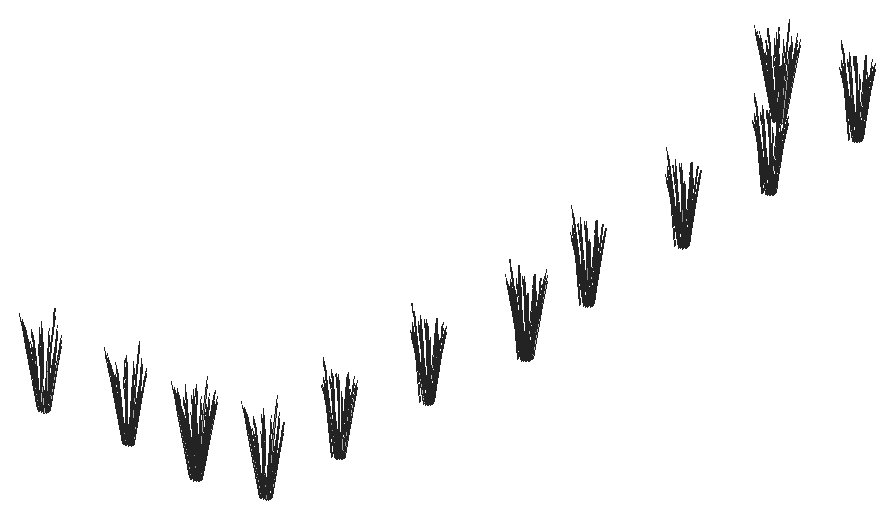
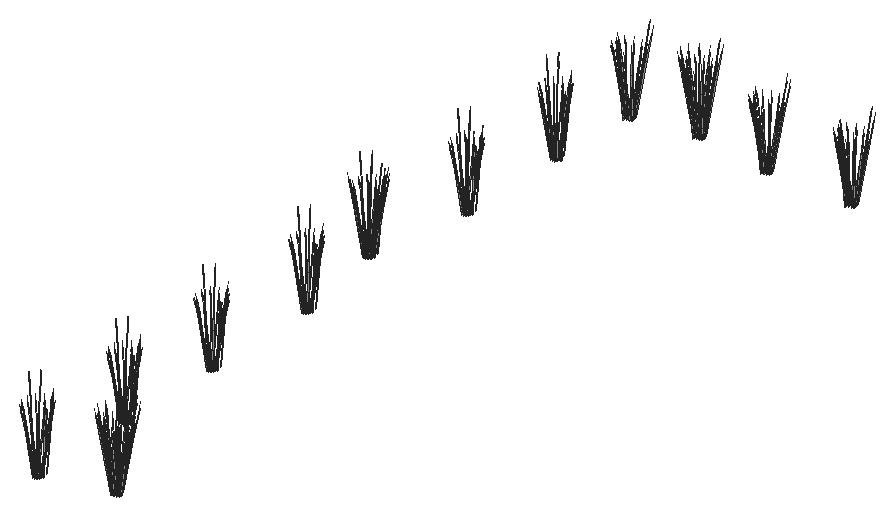
# SketchUp Ruby script. Lengths in inches.
U = 1.inch
M = Sketchup.active_model
def pt(a) = Geom::Point3d.new(a.map { |v| v * U })
def face(e, loops, mat)
  f = e.add_face(loops[0].map { |a| pt(a) })
  loops[1..].each { |l| e.add_face(l.map { |a| pt(a) }).erase! }
  f.material = f.back_material = mat if mat
  f
end
# faces: each face lists its corners as indices into pts; further lists are holes
def faces(e, pts, list, mat = nil) = list.each { |f| face(e, (f[0].is_a?(Array) ? f : [f]).map { |l| l.map { |i| pts[i] } }, mat) }
# xy, xz, yz: faces in a plane at the given z, y or x. An outline is a flat list of corners, or four numbers for a rectangle; further outlines are holes
def ring(l) = l.size == 4 ? [[l[0], l[1]], [l[2], l[1]], [l[2], l[3]], [l[0], l[3]]] : l.each_slice(2).to_a
def flat(e, list, mat, &to3) = list.each { |f| face(e, (f[0].is_a?(Array) ? f : [f]).map { |l| ring(l).map { |u, v| to3.(u, v) } }, mat) }
def xy(e, z, list, mat = nil) = flat(e, list, mat) { |x, y| [x, y, z] }
def xz(e, y, list, mat = nil) = flat(e, list, mat) { |x, z| [x, y, z] }
def yz(e, x, list, mat = nil) = flat(e, list, mat) { |y, z| [x, y, z] }
def lines(e, pts, list) = list.each { |a, b| e.add_line(pt(pts[a]), pt(pts[b])) }
# prism: a flat outline (further loops are holes) pulled along v
def prism(e, loops, v, mat = nil)
  f = face(e, loops, mat); d = Geom::Vector3d.new(v.map { |x| x * U })
  f.pushpull(f.normal.samedirection?(d) ? d.length : -d.length)
end
def box(e, o, s, mat = nil) = prism(e, [[o, [o[0] + s[0], o[1], o[2]], [o[0] + s[0], o[1] + s[1], o[2]], [o[0], o[1] + s[1], o[2]]]], [0, 0, s[2]], mat)
def at(x, y, z, deg = 0) = Geom::Transformation.translation(pt([x, y, z])) * Geom::Transformation.rotation(ORIGIN, Z_AXIS, deg.degrees)
def axes(o, x, y, z) = Geom::Transformation.new([*x, 0, *y, 0, *z, 0, *pt(o).to_a, 1])
def part(name) = M.definitions.add(name)
# library, detail: a bought-in or finely detailed component or shape, given as its bounding box
def library(name, o, s) = part(name).tap { |d| box(d.entities, o, s) }
def detail(e, o, s) = box(e.add_group.entities, o, s)
def put(e, d, t, mat = nil) = e.add_instance(d, t).tap { |i| i.material = mat if mat }
def group(e, t, mat = nil) = e.add_group.tap { |g| g.transformation = t; g.material = mat if mat }.entities
root = M.entities
M.materials.add("LightPink_Translucent").color = [175, 214, 192]
M.materials["LightPink_Translucent"].alpha = 0.75
c1 = part("blade")
p = [[2.15,0.21,22],[0,0.17,0],[0.09,0.45,0],[2.18,0.31,22],[2.29,0.31,22],[0.38,0.45,0],
  [2.48,0.24,33],[2.49,0.24,33],[2.48,0.22,33]]
faces(c1.entities,p,[[0,1,2,3],[4,5,2,3],[6,3,4,7],[8,0,3,6]])
c2 = part("seeds")
p = [[0.3,-0.1,1.38],[-0.01,-0.03,1.59],[-0.01,-0.03,0.03],[0.14,-0.07,-0.07],[0.29,-0.03,3],[0.15,0.01,3.11]]
faces(c2.entities,p,[[0,1,2,3],[1,0,4,5]],"LightPink_Translucent")
c3 = part("blade with seeds")
put(c3.entities,c1,at(0,0,0))
put(c3.entities,c2,axes([2.4,0.25,30.99],[1.5799,-0.05474,1.17369],[-0.12525,1.92788,0.29478],[-0.07173,-0.02425,1.56792]))
put(root,c3,axes([499.79,369.26,141.57],[0.40986,-0.11853,0.43682],[0.07113,0.46497,0.36018],[-0.09639,-0.13704,0.9039]))
put(root,c3,axes([498.96,369.9375,141.57],[0.30385,-0.34034,0.43682],[0.26205,0.36143,0.36018],[-0.14256,-0.06278,0.9039]))
put(root,c3,axes([501.97,372.85,141.57],[-0.30385,0.34034,0.43682],[-0.26205,-0.36143,0.36018],[0.14256,0.06278,0.9039]))
put(root,c3,axes([500.8,369.15,141.57],[0.40605,0.13503,0.43682],[-0.13885,0.44393,0.36018],[-0.0244,-0.17458,0.9039]))
put(root,c3,axes([501.14,373.53,141.57],[-0.40986,0.11853,0.43682],[-0.07113,-0.46497,0.36018],[0.09639,0.13704,0.9039]))
put(root,c3,axes([498.625,372.18,141.57],[-0.1022,-0.47536,0.43682],[0.4009,-0.0825,0.36018],[-0.11815,0.1118,0.9039]))
put(root,c3,axes([463.68,229.6,141.57],[0.47094,0.11642,0.43682],[-0.16104,0.38276,0.36018],[-0.0283,-0.15052,0.9039]))
put(root,c3,axes([465.05,232.79,141.57],[-0.35241,0.29344,0.43682],[-0.30393,-0.31162,0.36018],[0.16534,0.05413,0.9039]))
put(root,c3,axes([465.54,231.87,141.57],[-0.13503,0.40605,0.43682],[-0.44393,-0.13885,0.36018],[0.17458,-0.0244,0.9039]))
put(root,c3,axes([461.16,232.21,141.57],[-0.11853,-0.40986,0.43682],[0.46497,-0.07113,0.36018],[-0.13704,0.09639,0.9039]))
put(root,c3,axes([461.84,233.04,141.57],[-0.34034,-0.30385,0.43682],[0.36143,-0.26205,0.36018],[-0.06278,0.14256,0.9039]))
put(root,c3,axes([464.75,230.03,141.57],[0.34034,0.30385,0.43682],[-0.36143,0.26205,0.36018],[0.06278,-0.14256,0.9039]))
put(root,c3,axes([461.06,231.2,141.57],[0.13503,-0.40605,0.43682],[0.44393,0.13885,0.36018],[-0.17458,0.0244,0.9039]))
put(root,c3,axes([465.43,230.86,141.57],[0.11853,0.40986,0.43682],[-0.46497,0.07113,0.36018],[0.13704,-0.09639,0.9039]))
put(root,c3,axes([464.08,233.375,141.57],[-0.47536,0.1022,0.43682],[-0.0825,-0.4009,0.36018],[0.1118,0.11815,0.9039]))
put(root,c3,axes([463.68,558.11,141.57],[0.47094,0.11642,0.43682],[-0.16104,0.38276,0.36018],[-0.0283,-0.15052,0.9039]))
put(root,c3,axes([465.05,561.3,141.57],[-0.35241,0.29344,0.43682],[-0.30393,-0.31162,0.36018],[0.16534,0.05413,0.9039]))
put(root,c3,axes([465.54,560.38,141.57],[-0.13503,0.40605,0.43682],[-0.44393,-0.13885,0.36018],[0.17458,-0.0244,0.9039]))
put(root,c3,axes([461.16,560.73,141.57],[-0.11853,-0.40986,0.43682],[0.46497,-0.07113,0.36018],[-0.13704,0.09639,0.9039]))
put(root,c3,axes([461.84,561.56,141.57],[-0.34034,-0.30385,0.43682],[0.36143,-0.26205,0.36018],[-0.06278,0.14256,0.9039]))
put(root,c3,axes([464.75,558.54,141.57],[0.34034,0.30385,0.43682],[-0.36143,0.26205,0.36018],[0.06278,-0.14256,0.9039]))
put(root,c3,axes([461.06,559.71,141.57],[0.13503,-0.40605,0.43682],[0.44393,0.13885,0.36018],[-0.17458,0.0244,0.9039]))
put(root,c3,axes([465.43,559.37,141.57],[0.11853,0.40986,0.43682],[-0.46497,0.07113,0.36018],[0.13704,-0.09639,0.9039]))
put(root,c3,axes([464.08,561.89,141.57],[-0.47536,0.1022,0.43682],[-0.0825,-0.4009,0.36018],[0.1118,0.11815,0.9039]))
put(root,c3,axes([390.43,238,141.77],[0.14409,-0.34247,0.32227],[0.42037,0.09989,-0.41605],[0.03855,0.13788,0.79608]))
put(root,c3,axes([391.2,234.7,141.77],[-0.14409,0.34247,0.32227],[-0.42037,-0.09989,-0.41605],[-0.03855,-0.13788,0.79608]))
put(root,c3,axes([392.28,237.46,141.77],[-0.27194,-0.27882,0.32227],[0.31051,-0.26394,-0.41605],[0.15777,0.04016,0.79608]))
put(root,c3,axes([392.73,236.68,141.77],[-0.3972,-0.12423,0.32227],[0.11585,-0.36244,-0.41605],[0.15992,-0.03323,0.79608]))
put(root,c3,axes([389.35,235.24,141.77],[0.27194,0.27882,0.32227],[-0.31051,0.26394,-0.41605],[-0.15777,-0.04016,0.79608]))
put(root,c3,axes([389.53,237.62,141.77],[0.32338,-0.23447,0.32227],[0.30612,0.26773,-0.41605],[-0.04658,0.13603,0.79608]))
put(root,c3,axes([388.97,236.89,141.77],[0.41603,-0.06364,0.32227],[0.10985,0.36383,-0.41605],[-0.11922,0.09772,0.79608]))
put(root,c3,axes([391.44,237.95,141.77],[-0.07382,-0.3587,0.32227],[0.42197,-0.09472,-0.41605],[0.11334,0.10279,0.79608]))
put(root,c3,axes([392.67,235.8125,141.77],[-0.41603,0.06364,0.32227],[-0.10985,-0.36383,-0.41605],[0.11922,-0.09772,0.79608]))
put(root,c3,axes([388.9,236.02,141.77],[0.3972,0.12423,0.32227],[-0.11585,0.36244,-0.41605],[-0.15992,0.03323,0.79608]))
put(root,c3,axes([392.1,235.09,141.77],[-0.32338,0.23447,0.32227],[-0.30612,-0.26773,-0.41605],[0.04658,-0.13603,0.79608]))
put(root,c3,axes([390.1875,234.76,141.77],[0.07382,0.3587,0.32227],[-0.42197,0.09472,-0.41605],[-0.11334,-0.10279,0.79608]))
put(root,c3,axes([428.63,238,141.77],[0.14409,-0.34247,0.32227],[0.42037,0.09989,-0.41605],[0.03855,0.13788,0.79608]))
put(root,c3,axes([429.39,234.7,141.77],[-0.14409,0.34247,0.32227],[-0.42037,-0.09989,-0.41605],[-0.03855,-0.13788,0.79608]))
put(root,c3,axes([430.48,237.46,141.77],[-0.27194,-0.27882,0.32227],[0.31051,-0.26394,-0.41605],[0.15777,0.04016,0.79608]))
put(root,c3,axes([430.93,236.68,141.77],[-0.3972,-0.12423,0.32227],[0.11585,-0.36244,-0.41605],[0.15992,-0.03323,0.79608]))
put(root,c3,axes([427.54,235.24,141.77],[0.27194,0.27882,0.32227],[-0.31051,0.26394,-0.41605],[-0.15777,-0.04016,0.79608]))
put(root,c3,axes([427.72,237.62,141.77],[0.32338,-0.23447,0.32227],[0.30612,0.26773,-0.41605],[-0.04658,0.13603,0.79608]))
put(root,c3,axes([427.16,236.89,141.77],[0.41603,-0.06364,0.32227],[0.10985,0.36383,-0.41605],[-0.11922,0.09772,0.79608]))
put(root,c3,axes([429.64,237.95,141.77],[-0.07382,-0.3587,0.32227],[0.42197,-0.09472,-0.41605],[0.11334,0.10279,0.79608]))
put(root,c3,axes([430.86,235.8125,141.77],[-0.41603,0.06364,0.32227],[-0.10985,-0.36383,-0.41605],[0.11922,-0.09772,0.79608]))
put(root,c3,axes([427.09,236.02,141.77],[0.3972,0.12423,0.32227],[-0.11585,0.36244,-0.41605],[-0.15992,0.03323,0.79608]))
put(root,c3,axes([430.3,235.09,141.77],[-0.32338,0.23447,0.32227],[-0.30612,-0.26773,-0.41605],[0.04658,-0.13603,0.79608]))
put(root,c3,axes([428.38,234.76,141.77],[0.07382,0.3587,0.32227],[-0.42197,0.09472,-0.41605],[-0.11334,-0.10279,0.79608]))
put(root,c3,axes([490.64,238,141.77],[0.14409,-0.34247,0.32227],[0.42037,0.09989,-0.41605],[0.03855,0.13788,0.79608]))
put(root,c3,axes([491.4,234.7,141.77],[-0.14409,0.34247,0.32227],[-0.42037,-0.09989,-0.41605],[-0.03855,-0.13788,0.79608]))
put(root,c3,axes([492.49,237.46,141.77],[-0.27194,-0.27882,0.32227],[0.31051,-0.26394,-0.41605],[0.15777,0.04016,0.79608]))
put(root,c3,axes([492.9375,236.68,141.77],[-0.3972,-0.12423,0.32227],[0.11585,-0.36244,-0.41605],[0.15992,-0.03323,0.79608]))
put(root,c3,axes([489.55,235.24,141.77],[0.27194,0.27882,0.32227],[-0.31051,0.26394,-0.41605],[-0.15777,-0.04016,0.79608]))
put(root,c3,axes([489.73,237.62,141.77],[0.32338,-0.23447,0.32227],[0.30612,0.26773,-0.41605],[-0.04658,0.13603,0.79608]))
put(root,c3,axes([489.17,236.89,141.77],[0.41603,-0.06364,0.32227],[0.10985,0.36383,-0.41605],[-0.11922,0.09772,0.79608]))
put(root,c3,axes([491.65,237.95,141.77],[-0.07382,-0.3587,0.32227],[0.42197,-0.09472,-0.41605],[0.11334,0.10279,0.79608]))
put(root,c3,axes([492.87,235.8125,141.77],[-0.41603,0.06364,0.32227],[-0.10985,-0.36383,-0.41605],[0.11922,-0.09772,0.79608]))
put(root,c3,axes([489.11,236.02,141.77],[0.3972,0.12423,0.32227],[-0.11585,0.36244,-0.41605],[-0.15992,0.03323,0.79608]))
put(root,c3,axes([492.31,235.09,141.77],[-0.32338,0.23447,0.32227],[-0.30612,-0.26773,-0.41605],[0.04658,-0.13603,0.79608]))
put(root,c3,axes([490.39,234.76,141.77],[0.07382,0.3587,0.32227],[-0.42197,0.09472,-0.41605],[-0.11334,-0.10279,0.79608]))
put(root,c3,axes([491.37,275.12,141.77],[0.34247,0.14409,0.32227],[-0.09989,0.42037,-0.41605],[-0.13788,0.03855,0.79608]))
put(root,c3,axes([494.67,275.88,141.77],[-0.34247,-0.14409,0.32227],[0.09989,-0.42037,-0.41605],[0.13788,-0.03855,0.79608]))
put(root,c3,axes([491.91,276.97,141.77],[0.27882,-0.27194,0.32227],[0.26394,0.31051,-0.41605],[-0.04016,0.15777,0.79608]))
put(root,c3,axes([492.69,277.42,141.77],[0.12423,-0.3972,0.32227],[0.36244,0.11585,-0.41605],[0.03323,0.15992,0.79608]))
put(root,c3,axes([494.13,274.03,141.77],[-0.27882,0.27194,0.32227],[-0.26394,-0.31051,-0.41605],[0.04016,-0.15777,0.79608]))
put(root,c3,axes([491.76,274.21,141.77],[0.23447,0.32338,0.32227],[-0.26773,0.30612,-0.41605],[-0.13603,-0.04658,0.79608]))
put(root,c3,axes([492.48,273.65,141.77],[0.06364,0.41603,0.32227],[-0.36383,0.10985,-0.41605],[-0.09772,-0.11922,0.79608]))
put(root,c3,axes([491.43,276.13,141.77],[0.3587,-0.07382,0.32227],[0.09472,0.42197,-0.41605],[-0.10279,0.11334,0.79608]))
put(root,c3,axes([493.5625,277.35,141.77],[-0.06364,-0.41603,0.32227],[0.36383,-0.10985,-0.41605],[0.09772,0.11922,0.79608]))
put(root,c3,axes([493.35,273.59,141.77],[-0.12423,0.3972,0.32227],[-0.36244,-0.11585,-0.41605],[-0.03323,-0.15992,0.79608]))
put(root,c3,axes([494.29,276.79,141.77],[-0.23447,-0.32338,0.32227],[0.26773,-0.30612,-0.41605],[0.13603,0.04658,0.79608]))
put(root,c3,axes([494.62,274.875,141.77],[-0.3587,0.07382,0.32227],[-0.09472,-0.42197,-0.41605],[0.10279,-0.11334,0.79608]))
put(root,c3,axes([491.37,325.11,141.77],[0.34247,0.14409,0.32227],[-0.09989,0.42037,-0.41605],[-0.13788,0.03855,0.79608]))
put(root,c3,axes([494.67,325.87,141.77],[-0.34247,-0.14409,0.32227],[0.09989,-0.42037,-0.41605],[0.13788,-0.03855,0.79608]))
put(root,c3,axes([491.91,326.96,141.77],[0.27882,-0.27194,0.32227],[0.26394,0.31051,-0.41605],[-0.04016,0.15777,0.79608]))
put(root,c3,axes([492.69,327.4,141.77],[0.12423,-0.3972,0.32227],[0.36244,0.11585,-0.41605],[0.03323,0.15992,0.79608]))
put(root,c3,axes([494.13,324.02,141.77],[-0.27882,0.27194,0.32227],[-0.26394,-0.31051,-0.41605],[0.04016,-0.15777,0.79608]))
put(root,c3,axes([491.76,324.2,141.77],[0.23447,0.32338,0.32227],[-0.26773,0.30612,-0.41605],[-0.13603,-0.04658,0.79608]))
put(root,c3,axes([492.48,323.64,141.77],[0.06364,0.41603,0.32227],[-0.36383,0.10985,-0.41605],[-0.09772,-0.11922,0.79608]))
put(root,c3,axes([491.43,326.12,141.77],[0.3587,-0.07382,0.32227],[0.09472,0.42197,-0.41605],[-0.10279,0.11334,0.79608]))
put(root,c3,axes([493.5625,327.34,141.77],[-0.06364,-0.41603,0.32227],[0.36383,-0.10985,-0.41605],[0.09772,0.11922,0.79608]))
put(root,c3,axes([493.35,323.57,141.77],[-0.12423,0.3972,0.32227],[-0.36244,-0.11585,-0.41605],[-0.03323,-0.15992,0.79608]))
put(root,c3,axes([494.29,326.78,141.77],[-0.23447,-0.32338,0.32227],[0.26773,-0.30612,-0.41605],[0.13603,0.04658,0.79608]))
put(root,c3,axes([494.62,324.86,141.77],[-0.3587,0.07382,0.32227],[-0.09472,-0.42197,-0.41605],[0.10279,-0.11334,0.79608]))
put(root,c3,axes([491.37,415.23,141.77],[0.34247,0.14409,0.32227],[-0.09989,0.42037,-0.41605],[-0.13788,0.03855,0.79608]))
put(root,c3,axes([494.67,415.99,141.77],[-0.34247,-0.14409,0.32227],[0.09989,-0.42037,-0.41605],[0.13788,-0.03855,0.79608]))
put(root,c3,axes([491.91,417.08,141.77],[0.27882,-0.27194,0.32227],[0.26394,0.31051,-0.41605],[-0.04016,0.15777,0.79608]))
put(root,c3,axes([492.69,417.52,141.77],[0.12423,-0.3972,0.32227],[0.36244,0.11585,-0.41605],[0.03323,0.15992,0.79608]))
put(root,c3,axes([494.13,414.14,141.77],[-0.27882,0.27194,0.32227],[-0.26394,-0.31051,-0.41605],[0.04016,-0.15777,0.79608]))
put(root,c3,axes([491.76,414.32,141.77],[0.23447,0.32338,0.32227],[-0.26773,0.30612,-0.41605],[-0.13603,-0.04658,0.79608]))
put(root,c3,axes([492.48,413.76,141.77],[0.06364,0.41603,0.32227],[-0.36383,0.10985,-0.41605],[-0.09772,-0.11922,0.79608]))
put(root,c3,axes([491.43,416.24,141.77],[0.3587,-0.07382,0.32227],[0.09472,0.42197,-0.41605],[-0.10279,0.11334,0.79608]))
put(root,c3,axes([493.5625,417.46,141.77],[-0.06364,-0.41603,0.32227],[0.36383,-0.10985,-0.41605],[0.09772,0.11922,0.79608]))
put(root,c3,axes([493.35,413.69,141.77],[-0.12423,0.3972,0.32227],[-0.36244,-0.11585,-0.41605],[-0.03323,-0.15992,0.79608]))
put(root,c3,axes([494.29,416.9,141.77],[-0.23447,-0.32338,0.32227],[0.26773,-0.30612,-0.41605],[0.13603,0.04658,0.79608]))
put(root,c3,axes([494.62,414.98,141.77],[-0.3587,0.07382,0.32227],[-0.09472,-0.42197,-0.41605],[0.10279,-0.11334,0.79608]))
put(root,c3,axes([491.37,468.8,141.77],[0.34247,0.14409,0.32227],[-0.09989,0.42037,-0.41605],[-0.13788,0.03855,0.79608]))
put(root,c3,axes([494.67,469.5625,141.77],[-0.34247,-0.14409,0.32227],[0.09989,-0.42037,-0.41605],[0.13788,-0.03855,0.79608]))
put(root,c3,axes([491.91,470.65,141.77],[0.27882,-0.27194,0.32227],[0.26394,0.31051,-0.41605],[-0.04016,0.15777,0.79608]))
put(root,c3,axes([492.69,471.1,141.77],[0.12423,-0.3972,0.32227],[0.36244,0.11585,-0.41605],[0.03323,0.15992,0.79608]))
put(root,c3,axes([494.13,467.71,141.77],[-0.27882,0.27194,0.32227],[-0.26394,-0.31051,-0.41605],[0.04016,-0.15777,0.79608]))
put(root,c3,axes([491.76,467.89,141.77],[0.23447,0.32338,0.32227],[-0.26773,0.30612,-0.41605],[-0.13603,-0.04658,0.79608]))
put(root,c3,axes([492.48,467.33,141.77],[0.06364,0.41603,0.32227],[-0.36383,0.10985,-0.41605],[-0.09772,-0.11922,0.79608]))
put(root,c3,axes([491.43,469.81,141.77],[0.3587,-0.07382,0.32227],[0.09472,0.42197,-0.41605],[-0.10279,0.11334,0.79608]))
put(root,c3,axes([493.5625,471.03,141.77],[-0.06364,-0.41603,0.32227],[0.36383,-0.10985,-0.41605],[0.09772,0.11922,0.79608]))
put(root,c3,axes([493.35,467.27,141.77],[-0.12423,0.3972,0.32227],[-0.36244,-0.11585,-0.41605],[-0.03323,-0.15992,0.79608]))
put(root,c3,axes([494.29,470.47,141.77],[-0.23447,-0.32338,0.32227],[0.26773,-0.30612,-0.41605],[0.13603,0.04658,0.79608]))
put(root,c3,axes([494.62,468.55,141.77],[-0.3587,0.07382,0.32227],[-0.09472,-0.42197,-0.41605],[0.10279,-0.11334,0.79608]))
put(root,c3,axes([491.37,518.01,141.77],[0.34247,0.14409,0.32227],[-0.09989,0.42037,-0.41605],[-0.13788,0.03855,0.79608]))
put(root,c3,axes([494.67,518.77,141.77],[-0.34247,-0.14409,0.32227],[0.09989,-0.42037,-0.41605],[0.13788,-0.03855,0.79608]))
put(root,c3,axes([491.91,519.86,141.77],[0.27882,-0.27194,0.32227],[0.26394,0.31051,-0.41605],[-0.04016,0.15777,0.79608]))
put(root,c3,axes([492.69,520.31,141.77],[0.12423,-0.3972,0.32227],[0.36244,0.11585,-0.41605],[0.03323,0.15992,0.79608]))
put(root,c3,axes([494.13,516.92,141.77],[-0.27882,0.27194,0.32227],[-0.26394,-0.31051,-0.41605],[0.04016,-0.15777,0.79608]))
put(root,c3,axes([491.76,517.1,141.77],[0.23447,0.32338,0.32227],[-0.26773,0.30612,-0.41605],[-0.13603,-0.04658,0.79608]))
put(root,c3,axes([492.48,516.54,141.77],[0.06364,0.41603,0.32227],[-0.36383,0.10985,-0.41605],[-0.09772,-0.11922,0.79608]))
put(root,c3,axes([491.43,519.02,141.77],[0.3587,-0.07382,0.32227],[0.09472,0.42197,-0.41605],[-0.10279,0.11334,0.79608]))
put(root,c3,axes([493.5625,520.24,141.77],[-0.06364,-0.41603,0.32227],[0.36383,-0.10985,-0.41605],[0.09772,0.11922,0.79608]))
put(root,c3,axes([493.35,516.48,141.77],[-0.12423,0.3972,0.32227],[-0.36244,-0.11585,-0.41605],[-0.03323,-0.15992,0.79608]))
put(root,c3,axes([494.29,519.68,141.77],[-0.23447,-0.32338,0.32227],[0.26773,-0.30612,-0.41605],[0.13603,0.04658,0.79608]))
put(root,c3,axes([494.62,517.76,141.77],[-0.3587,0.07382,0.32227],[-0.09472,-0.42197,-0.41605],[0.10279,-0.11334,0.79608]))
put(root,c3,axes([491.37,567.06,141.77],[0.34247,0.14409,0.32227],[-0.09989,0.42037,-0.41605],[-0.13788,0.03855,0.79608]))
put(root,c3,axes([494.67,567.82,141.77],[-0.34247,-0.14409,0.32227],[0.09989,-0.42037,-0.41605],[0.13788,-0.03855,0.79608]))
put(root,c3,axes([491.91,568.91,141.77],[0.27882,-0.27194,0.32227],[0.26394,0.31051,-0.41605],[-0.04016,0.15777,0.79608]))
put(root,c3,axes([492.69,569.36,141.77],[0.12423,-0.3972,0.32227],[0.36244,0.11585,-0.41605],[0.03323,0.15992,0.79608]))
put(root,c3,axes([494.13,565.97,141.77],[-0.27882,0.27194,0.32227],[-0.26394,-0.31051,-0.41605],[0.04016,-0.15777,0.79608]))
put(root,c3,axes([491.76,566.15,141.77],[0.23447,0.32338,0.32227],[-0.26773,0.30612,-0.41605],[-0.13603,-0.04658,0.79608]))
put(root,c3,axes([492.48,565.59,141.77],[0.06364,0.41603,0.32227],[-0.36383,0.10985,-0.41605],[-0.09772,-0.11922,0.79608]))
put(root,c3,axes([491.43,568.07,141.77],[0.3587,-0.07382,0.32227],[0.09472,0.42197,-0.41605],[-0.10279,0.11334,0.79608]))
put(root,c3,axes([493.5625,569.29,141.77],[-0.06364,-0.41603,0.32227],[0.36383,-0.10985,-0.41605],[0.09772,0.11922,0.79608]))
put(root,c3,axes([493.35,565.52,141.77],[-0.12423,0.3972,0.32227],[-0.36244,-0.11585,-0.41605],[-0.03323,-0.15992,0.79608]))
put(root,c3,axes([494.29,568.73,141.77],[-0.23447,-0.32338,0.32227],[0.26773,-0.30612,-0.41605],[0.13603,0.04658,0.79608]))
put(root,c3,axes([494.62,566.8125,141.77],[-0.3587,0.07382,0.32227],[-0.09472,-0.42197,-0.41605],[0.10279,-0.11334,0.79608]))
put(root,c3,axes([498.8125,371.01,141.86],[0.34247,0.14409,0.32227],[-0.09989,0.42037,-0.41605],[-0.13788,0.03855,0.79608]))
put(root,c3,axes([502.12,371.78,141.86],[-0.34247,-0.14409,0.32227],[0.09989,-0.42037,-0.41605],[0.13788,-0.03855,0.79608]))
put(root,c3,axes([499.35,372.86,141.86],[0.27882,-0.27194,0.32227],[0.26394,0.31051,-0.41605],[-0.04016,0.15777,0.79608]))
put(root,c3,axes([500.14,373.3125,141.86],[0.12423,-0.3972,0.32227],[0.36244,0.11585,-0.41605],[0.03323,0.15992,0.79608]))
put(root,c3,axes([501.58,369.93,141.86],[-0.27882,0.27194,0.32227],[-0.26394,-0.31051,-0.41605],[0.04016,-0.15777,0.79608]))
put(root,c3,axes([499.2,370.11,141.86],[0.23447,0.32338,0.32227],[-0.26773,0.30612,-0.41605],[-0.13603,-0.04658,0.79608]))
put(root,c3,axes([499.92,369.55,141.86],[0.06364,0.41603,0.32227],[-0.36383,0.10985,-0.41605],[-0.09772,-0.11922,0.79608]))
put(root,c3,axes([498.87,372.02,141.86],[0.3587,-0.07382,0.32227],[0.09472,0.42197,-0.41605],[-0.10279,0.11334,0.79608]))
put(root,c3,axes([501.01,373.24,141.86],[-0.06364,-0.41603,0.32227],[0.36383,-0.10985,-0.41605],[0.09772,0.11922,0.79608]))
put(root,c3,axes([500.79,369.48,141.86],[-0.12423,0.3972,0.32227],[-0.36244,-0.11585,-0.41605],[-0.03323,-0.15992,0.79608]))
put(root,c3,axes([501.73,372.68,141.86],[-0.23447,-0.32338,0.32227],[0.26773,-0.30612,-0.41605],[0.13603,0.04658,0.79608]))
put(root,c3,axes([502.06,370.77,141.86],[-0.3587,0.07382,0.32227],[-0.09472,-0.42197,-0.41605],[0.10279,-0.11334,0.79608]))
put(root,c3,axes([462.92,233.1875,141.86],[0.14409,-0.34247,0.32227],[0.42037,0.09989,-0.41605],[0.03855,0.13788,0.79608]))
put(root,c3,axes([463.68,229.88,141.86],[-0.14409,0.34247,0.32227],[-0.42037,-0.09989,-0.41605],[-0.03855,-0.13788,0.79608]))
put(root,c3,axes([464.77,232.65,141.86],[-0.27194,-0.27882,0.32227],[0.31051,-0.26394,-0.41605],[0.15777,0.04016,0.79608]))
put(root,c3,axes([465.21,231.86,141.86],[-0.3972,-0.12423,0.32227],[0.11585,-0.36244,-0.41605],[0.15992,-0.03323,0.79608]))
put(root,c3,axes([461.83,230.42,141.86],[0.27194,0.27882,0.32227],[-0.31051,0.26394,-0.41605],[-0.15777,-0.04016,0.79608]))
put(root,c3,axes([462.01,232.8,141.86],[0.32338,-0.23447,0.32227],[0.30612,0.26773,-0.41605],[-0.04658,0.13603,0.79608]))
put(root,c3,axes([461.45,232.08,141.86],[0.41603,-0.06364,0.32227],[0.10985,0.36383,-0.41605],[-0.11922,0.09772,0.79608]))
put(root,c3,axes([463.93,233.13,141.86],[-0.07382,-0.3587,0.32227],[0.42197,-0.09472,-0.41605],[0.11334,0.10279,0.79608]))
put(root,c3,axes([465.15,230.99,141.86],[-0.41603,0.06364,0.32227],[-0.10985,-0.36383,-0.41605],[0.11922,-0.09772,0.79608]))
put(root,c3,axes([461.38,231.21,141.86],[0.3972,0.12423,0.32227],[-0.11585,0.36244,-0.41605],[-0.15992,0.03323,0.79608]))
put(root,c3,axes([464.59,230.27,141.86],[-0.32338,0.23447,0.32227],[-0.30612,-0.26773,-0.41605],[0.04658,-0.13603,0.79608]))
put(root,c3,axes([462.67,229.94,141.86],[0.07382,0.3587,0.32227],[-0.42197,0.09472,-0.41605],[-0.11334,-0.10279,0.79608]))
put(root,c3,axes([462.92,561.7,141.86],[0.14409,-0.34247,0.32227],[0.42037,0.09989,-0.41605],[0.03855,0.13788,0.79608]))
put(root,c3,axes([463.68,558.4,141.86],[-0.14409,0.34247,0.32227],[-0.42037,-0.09989,-0.41605],[-0.03855,-0.13788,0.79608]))
put(root,c3,axes([464.77,561.16,141.86],[-0.27194,-0.27882,0.32227],[0.31051,-0.26394,-0.41605],[0.15777,0.04016,0.79608]))
put(root,c3,axes([465.21,560.375,141.86],[-0.3972,-0.12423,0.32227],[0.11585,-0.36244,-0.41605],[0.15992,-0.03323,0.79608]))
put(root,c3,axes([461.83,558.9375,141.86],[0.27194,0.27882,0.32227],[-0.31051,0.26394,-0.41605],[-0.15777,-0.04016,0.79608]))
put(root,c3,axes([462.01,561.3125,141.86],[0.32338,-0.23447,0.32227],[0.30612,0.26773,-0.41605],[-0.04658,0.13603,0.79608]))
put(root,c3,axes([461.45,560.59,141.86],[0.41603,-0.06364,0.32227],[0.10985,0.36383,-0.41605],[-0.11922,0.09772,0.79608]))
put(root,c3,axes([463.93,561.64,141.86],[-0.07382,-0.3587,0.32227],[0.42197,-0.09472,-0.41605],[0.11334,0.10279,0.79608]))
put(root,c3,axes([465.15,559.51,141.86],[-0.41603,0.06364,0.32227],[-0.10985,-0.36383,-0.41605],[0.11922,-0.09772,0.79608]))
put(root,c3,axes([461.38,559.72,141.86],[0.3972,0.12423,0.32227],[-0.11585,0.36244,-0.41605],[-0.15992,0.03323,0.79608]))
put(root,c3,axes([464.59,558.78,141.86],[-0.32338,0.23447,0.32227],[-0.30612,-0.26773,-0.41605],[0.04658,-0.13603,0.79608]))
put(root,c3,axes([462.67,558.45,141.86],[0.07382,0.3587,0.32227],[-0.42197,0.09472,-0.41605],[-0.11334,-0.10279,0.79608]))
put(root,c3,axes([390.43,238.29,141.78],[-0.47094,-0.11642,0.48487],[0.16104,-0.38276,0.3998],[0.0283,0.15052,1.00333]))
put(root,c3,axes([428.625,238.29,141.78],[-0.47094,-0.11642,0.48487],[0.16104,-0.38276,0.3998],[0.0283,0.15052,1.00333]))
put(root,c3,axes([490.63,238.29,141.78],[-0.47094,-0.11642,0.48487],[0.16104,-0.38276,0.3998],[0.0283,0.15052,1.00333]))
put(root,c3,axes([491.09,275.11,141.78],[0.11642,-0.47094,0.48487],[0.38276,0.16104,0.3998],[-0.15052,0.0283,1.00333]))
put(root,c3,axes([491.09,325.1,141.78],[0.11642,-0.47094,0.48487],[0.38276,0.16104,0.3998],[-0.15052,0.0283,1.00333]))
put(root,c3,axes([491.09,415.22,141.78],[0.11642,-0.47094,0.48487],[0.38276,0.16104,0.3998],[-0.15052,0.0283,1.00333]))
put(root,c3,axes([491.09,468.79,141.78],[0.11642,-0.47094,0.48487],[0.38276,0.16104,0.3998],[-0.15052,0.0283,1.00333]))
put(root,c3,axes([491.09,518,141.78],[0.11642,-0.47094,0.48487],[0.38276,0.16104,0.3998],[-0.15052,0.0283,1.00333]))
put(root,c3,axes([491.09,567.05,141.78],[0.11642,-0.47094,0.48487],[0.38276,0.16104,0.3998],[-0.15052,0.0283,1.00333]))
put(root,c3,axes([388.92,234.99,141.81],[0.3947,-0.32865,0.48924],[0.34041,0.34902,0.4034],[-0.18518,-0.06062,1.01237]))
put(root,c3,axes([390,234.34,141.81],[0.53241,-0.11446,0.48924],[0.0924,0.44901,0.4034],[-0.12521,-0.13233,1.01237]))
put(root,c3,axes([427.12,234.99,141.81],[0.3947,-0.32865,0.48924],[0.34041,0.34902,0.4034],[-0.18518,-0.06062,1.01237]))
put(root,c3,axes([428.19,234.34,141.81],[0.53241,-0.11446,0.48924],[0.0924,0.44901,0.4034],[-0.12521,-0.13233,1.01237]))
put(root,c3,axes([489.125,234.99,141.81],[0.3947,-0.32865,0.48924],[0.34041,0.34902,0.4034],[-0.18518,-0.06062,1.01237]))
put(root,c3,axes([490.2,234.34,141.81],[0.53241,-0.11446,0.48924],[0.0924,0.44901,0.4034],[-0.12521,-0.13233,1.01237]))
put(root,c3,axes([494.38,273.61,141.81],[0.32865,0.3947,0.48924],[-0.34902,0.34041,0.4034],[0.06062,-0.18518,1.01237]))
put(root,c3,axes([495.04,274.68,141.81],[0.11446,0.53241,0.48924],[-0.44901,0.0924,0.4034],[0.13233,-0.12521,1.01237]))
put(root,c3,axes([494.38,323.59,141.81],[0.32865,0.3947,0.48924],[-0.34902,0.34041,0.4034],[0.06062,-0.18518,1.01237]))
put(root,c3,axes([495.04,324.67,141.81],[0.11446,0.53241,0.48924],[-0.44901,0.0924,0.4034],[0.13233,-0.12521,1.01237]))
put(root,c3,axes([494.38,413.71,141.81],[0.32865,0.3947,0.48924],[-0.34902,0.34041,0.4034],[0.06062,-0.18518,1.01237]))
put(root,c3,axes([495.04,414.79,141.81],[0.11446,0.53241,0.48924],[-0.44901,0.0924,0.4034],[0.13233,-0.12521,1.01237]))
put(root,c3,axes([494.38,467.29,141.81],[0.32865,0.3947,0.48924],[-0.34902,0.34041,0.4034],[0.06062,-0.18518,1.01237]))
put(root,c3,axes([495.04,468.36,141.81],[0.11446,0.53241,0.48924],[-0.44901,0.0924,0.4034],[0.13233,-0.12521,1.01237]))
put(root,c3,axes([494.38,516.5,141.81],[0.32865,0.3947,0.48924],[-0.34902,0.34041,0.4034],[0.06062,-0.18518,1.01237]))
put(root,c3,axes([495.04,517.57,141.81],[0.11446,0.53241,0.48924],[-0.44901,0.0924,0.4034],[0.13233,-0.12521,1.01237]))
put(root,c3,axes([494.38,565.54,141.81],[0.32865,0.3947,0.48924],[-0.34902,0.34041,0.4034],[0.06062,-0.18518,1.01237]))
put(root,c3,axes([495.04,566.62,141.81],[0.11446,0.53241,0.48924],[-0.44901,0.0924,0.4034],[0.13233,-0.12521,1.01237]))
put(root,c3,axes([498.53,371.01,141.87],[0.11642,-0.47094,0.48487],[0.38276,0.16104,0.3998],[-0.15052,0.0283,1.00333]))
put(root,c3,axes([462.91,233.47,141.87],[-0.47094,-0.11642,0.48487],[0.16104,-0.38276,0.3998],[0.0283,0.15052,1.00333]))
put(root,c3,axes([462.91,561.98,141.87],[-0.47094,-0.11642,0.48487],[0.16104,-0.38276,0.3998],[0.0283,0.15052,1.00333]))
put(root,c3,axes([501.83,369.5,141.9],[0.32865,0.3947,0.48924],[-0.34902,0.34041,0.4034],[0.06062,-0.18518,1.01237]))
put(root,c3,axes([502.48,370.58,141.9],[0.11446,0.53241,0.48924],[-0.44901,0.0924,0.4034],[0.13233,-0.12521,1.01237]))
put(root,c3,axes([461.4,230.17,141.9],[0.3947,-0.32865,0.48924],[0.34041,0.34902,0.4034],[-0.18518,-0.06062,1.01237]))
put(root,c3,axes([462.48,229.52,141.9],[0.53241,-0.11446,0.48924],[0.0924,0.44901,0.4034],[-0.12521,-0.13233,1.01237]))
put(root,c3,axes([461.4,558.6875,141.9],[0.3947,-0.32865,0.48924],[0.34041,0.34902,0.4034],[-0.18518,-0.06062,1.01237]))
put(root,c3,axes([462.48,558.03,141.9],[0.53241,-0.11446,0.48924],[0.0924,0.44901,0.4034],[-0.12521,-0.13233,1.01237]))
put(root,c3,axes([391,239.23,142.31],[0.33028,-0.25548,-0.05904],[0.30262,0.27981,-0.26768],[0.02131,0.07928,0.88292]))
put(root,c3,axes([388.02,237.93,142.31],[0.42175,0.11887,-0.05904],[-0.12974,0.36587,-0.26768],[-0.06898,0.05555,0.88292]))
put(root,c3,axes([429.19,239.23,142.31],[0.33028,-0.25548,-0.05904],[0.30262,0.27981,-0.26768],[0.02131,0.07928,0.88292]))
put(root,c3,axes([426.22,237.93,142.31],[0.42175,0.11887,-0.05904],[-0.12974,0.36587,-0.26768],[-0.06898,0.05555,0.88292]))
put(root,c3,axes([491.21,239.23,142.31],[0.33028,-0.25548,-0.05904],[0.30262,0.27981,-0.26768],[0.02131,0.07928,0.88292]))
put(root,c3,axes([488.23,237.93,142.31],[0.42175,0.11887,-0.05904],[-0.12974,0.36587,-0.26768],[-0.06898,0.05555,0.88292]))
put(root,c3,axes([490.15,275.69,142.31],[0.25548,0.33028,-0.05904],[-0.27981,0.30262,-0.26768],[-0.07928,0.02131,0.88292]))
put(root,c3,axes([491.45,272.71,142.31],[-0.11887,0.42175,-0.05904],[-0.36587,-0.12974,-0.26768],[-0.05555,-0.06898,0.88292]))
put(root,c3,axes([490.15,325.67,142.31],[0.25548,0.33028,-0.05904],[-0.27981,0.30262,-0.26768],[-0.07928,0.02131,0.88292]))
put(root,c3,axes([491.45,322.69,142.31],[-0.11887,0.42175,-0.05904],[-0.36587,-0.12974,-0.26768],[-0.05555,-0.06898,0.88292]))
put(root,c3,axes([490.15,415.79,142.31],[0.25548,0.33028,-0.05904],[-0.27981,0.30262,-0.26768],[-0.07928,0.02131,0.88292]))
put(root,c3,axes([491.45,412.8125,142.31],[-0.11887,0.42175,-0.05904],[-0.36587,-0.12974,-0.26768],[-0.05555,-0.06898,0.88292]))
put(root,c3,axes([490.15,469.37,142.31],[0.25548,0.33028,-0.05904],[-0.27981,0.30262,-0.26768],[-0.07928,0.02131,0.88292]))
put(root,c3,axes([491.45,466.39,142.31],[-0.11887,0.42175,-0.05904],[-0.36587,-0.12974,-0.26768],[-0.05555,-0.06898,0.88292]))
put(root,c3,axes([490.15,518.58,142.31],[0.25548,0.33028,-0.05904],[-0.27981,0.30262,-0.26768],[-0.07928,0.02131,0.88292]))
put(root,c3,axes([491.45,515.6,142.31],[-0.11887,0.42175,-0.05904],[-0.36587,-0.12974,-0.26768],[-0.05555,-0.06898,0.88292]))
put(root,c3,axes([490.15,567.625,142.31],[0.25548,0.33028,-0.05904],[-0.27981,0.30262,-0.26768],[-0.07928,0.02131,0.88292]))
put(root,c3,axes([491.45,564.65,142.31],[-0.11887,0.42175,-0.05904],[-0.36587,-0.12974,-0.26768],[-0.05555,-0.06898,0.88292]))
put(root,c3,axes([497.59,371.58,142.4],[0.25548,0.33028,-0.05904],[-0.27981,0.30262,-0.26768],[-0.07928,0.02131,0.88292]))
put(root,c3,axes([498.89,368.6,142.4],[-0.11887,0.42175,-0.05904],[-0.36587,-0.12974,-0.26768],[-0.05555,-0.06898,0.88292]))
put(root,c3,axes([463.48,234.41,142.4],[0.33028,-0.25548,-0.05904],[0.30262,0.27981,-0.26768],[0.02131,0.07928,0.88292]))
put(root,c3,axes([460.5,233.11,142.4],[0.42175,0.11887,-0.05904],[-0.12974,0.36587,-0.26768],[-0.06898,0.05555,0.88292]))
put(root,c3,axes([463.48,562.92,142.4],[0.33028,-0.25548,-0.05904],[0.30262,0.27981,-0.26768],[0.02131,0.07928,0.88292]))
put(root,c3,axes([460.5,561.62,142.4],[0.42175,0.11887,-0.05904],[-0.12974,0.36587,-0.26768],[-0.06898,0.05555,0.88292]))
